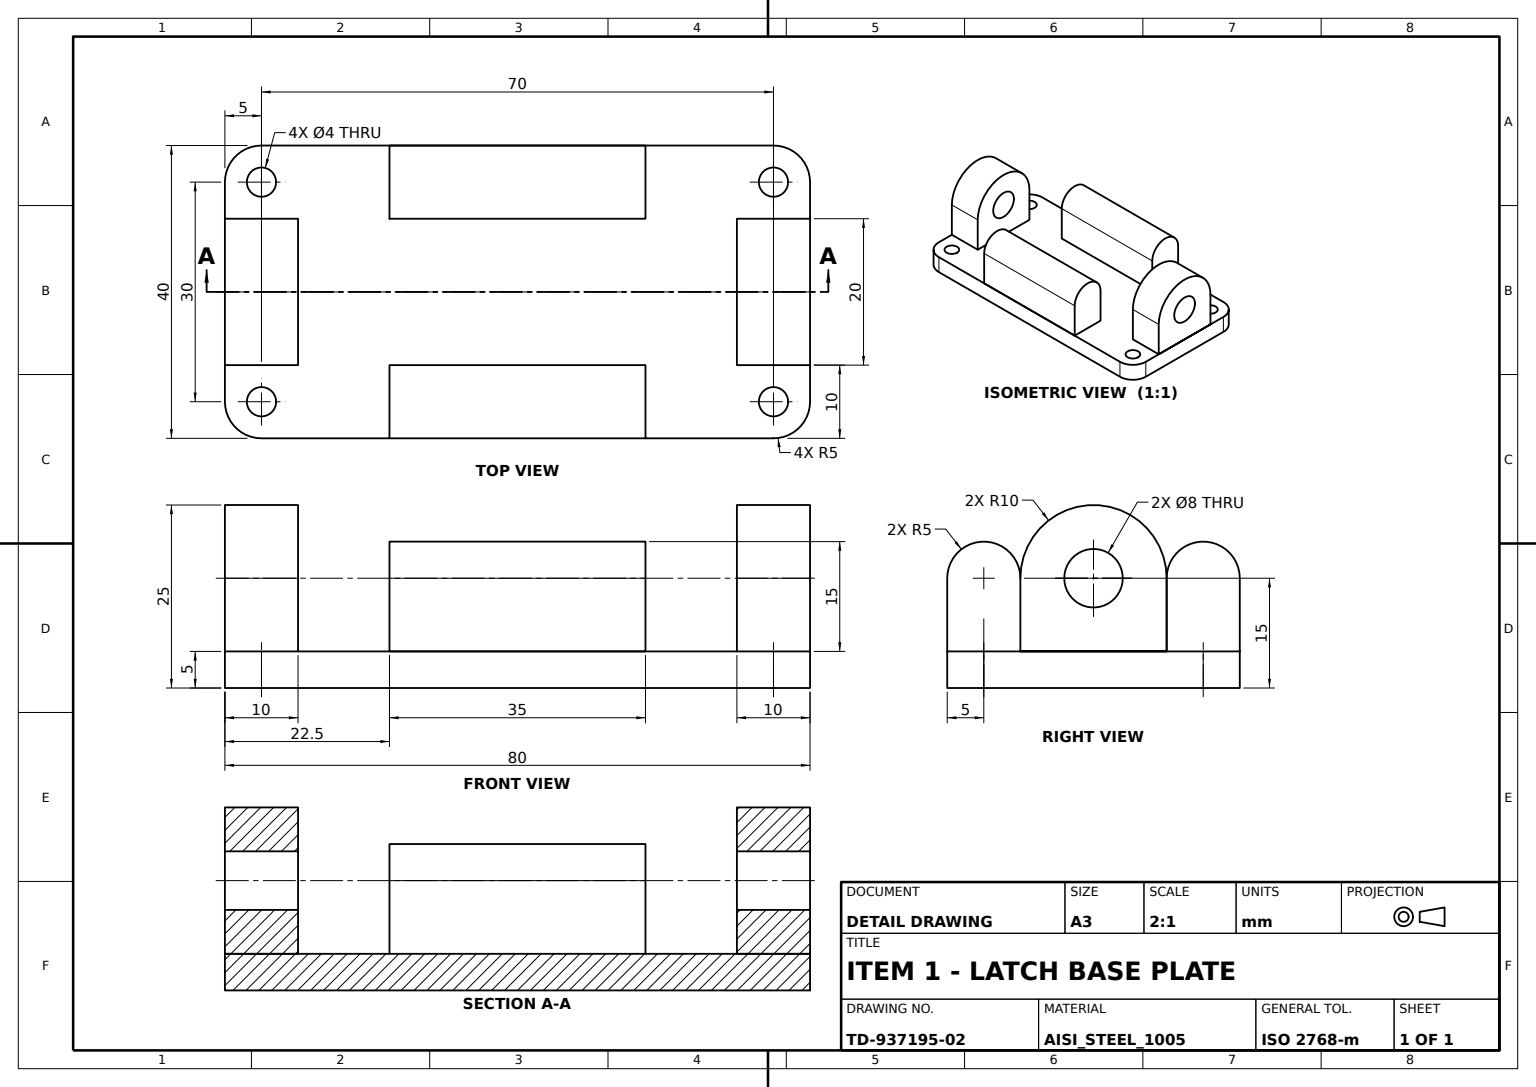
ISO-10303-21;
HEADER;
FILE_DESCRIPTION((''),'2;1');
FILE_NAME('','',(''),(''),'','','');
FILE_SCHEMA(('AUTOMOTIVE_DESIGN'));
ENDSEC;
DATA;
#1=APPLICATION_CONTEXT('');
#2=PRODUCT_CONTEXT('',#1,'mechanical');
#3=PRODUCT('','','',(#2));
#4=PRODUCT_DEFINITION_FORMATION('','',#3);
#5=PRODUCT_DEFINITION_CONTEXT('',#1,'design');
#6=PRODUCT_DEFINITION('','',#4,#5);
#7=PRODUCT_DEFINITION_SHAPE('','',#6);
#8=(LENGTH_UNIT()NAMED_UNIT(*)SI_UNIT(.MILLI.,.METRE.));
#9=(NAMED_UNIT(*)PLANE_ANGLE_UNIT()SI_UNIT($,.RADIAN.));
#10=(NAMED_UNIT(*)SI_UNIT($,.STERADIAN.)SOLID_ANGLE_UNIT());
#11=UNCERTAINTY_MEASURE_WITH_UNIT(LENGTH_MEASURE(0.005),#8,'distance_accuracy_value','');
#12=(GEOMETRIC_REPRESENTATION_CONTEXT(3)GLOBAL_UNCERTAINTY_ASSIGNED_CONTEXT((#11))GLOBAL_UNIT_ASSIGNED_CONTEXT((#8,#9,#10))REPRESENTATION_CONTEXT('',''));
#13=CARTESIAN_POINT('',(-17.5,10.,5.));
#14=VERTEX_POINT('',#13);
#15=CARTESIAN_POINT('',(17.5,10.,5.));
#16=VERTEX_POINT('',#15);
#17=DIRECTION('',(-1.,0.,0.));
#18=VECTOR('',#17,1000.);
#19=LINE('',#15,#18);
#20=EDGE_CURVE('',#14,#16,#19,.F.);
#21=ORIENTED_EDGE('',*,*,#20,.T.);
#22=CARTESIAN_POINT('',(17.5,10.,15.));
#23=VERTEX_POINT('',#22);
#24=CARTESIAN_POINT('',(17.5,10.,20.));
#25=DIRECTION('',(0.,0.,-1.));
#26=VECTOR('',#25,1000.);
#27=LINE('',#24,#26);
#28=EDGE_CURVE('',#16,#23,#27,.F.);
#29=ORIENTED_EDGE('',*,*,#28,.T.);
#30=CARTESIAN_POINT('',(-17.5,10.,15.));
#31=VERTEX_POINT('',#30);
#32=CARTESIAN_POINT('',(-20.5,10.,15.));
#33=DIRECTION('',(1.,0.,0.));
#34=VECTOR('',#33,1000.);
#35=LINE('',#32,#34);
#36=EDGE_CURVE('',#31,#23,#35,.T.);
#37=ORIENTED_EDGE('',*,*,#36,.F.);
#38=DIRECTION('',(0.,0.,1.));
#39=VECTOR('',#38,1000.);
#40=LINE('',#13,#39);
#41=EDGE_CURVE('',#31,#14,#40,.F.);
#42=ORIENTED_EDGE('',*,*,#41,.T.);
#43=EDGE_LOOP('',(#21,#29,#37,#42));
#44=FACE_BOUND('',#43,.T.);
#45=CARTESIAN_POINT('',(0.,10.,0.));
#46=DIRECTION('',(0.,1.,0.));
#47=AXIS2_PLACEMENT_3D('',#45,#46,#38);
#48=PLANE('',#47);
#49=ADVANCED_FACE('',(#44),#48,.F.);
#50=CARTESIAN_POINT('',(-17.5,20.,15.));
#51=VERTEX_POINT('',#50);
#52=CARTESIAN_POINT('',(17.5,20.,15.));
#53=VERTEX_POINT('',#52);
#54=CARTESIAN_POINT('',(-20.5,20.,15.));
#55=LINE('',#54,#34);
#56=EDGE_CURVE('',#51,#53,#55,.T.);
#57=ORIENTED_EDGE('',*,*,#56,.F.);
#58=CARTESIAN_POINT('',(-17.5,15.,15.));
#59=AXIS2_PLACEMENT_3D('',#58,#17,#38);
#60=CIRCLE('',#59,5.);
#61=EDGE_CURVE('',#31,#51,#60,.T.);
#62=ORIENTED_EDGE('',*,*,#61,.F.);
#63=ORIENTED_EDGE('',*,*,#36,.T.);
#64=CARTESIAN_POINT('',(17.5,15.,15.));
#65=DIRECTION('',(0.,-1.,0.));
#66=AXIS2_PLACEMENT_3D('',#64,#33,#65);
#67=CIRCLE('',#66,5.);
#68=EDGE_CURVE('',#53,#23,#67,.T.);
#69=ORIENTED_EDGE('',*,*,#68,.F.);
#70=EDGE_LOOP('',(#57,#62,#63,#69));
#71=FACE_BOUND('',#70,.T.);
#72=CARTESIAN_POINT('',(-20.5,15.,15.));
#73=AXIS2_PLACEMENT_3D('',#72,#33,#25);
#74=CYLINDRICAL_SURFACE('',#73,5.);
#75=ADVANCED_FACE('',(#71),#74,.T.);
#76=CARTESIAN_POINT('',(-17.5,20.,5.));
#77=VERTEX_POINT('',#76);
#78=VECTOR('',#46,1000.);
#79=LINE('',#13,#78);
#80=EDGE_CURVE('',#14,#77,#79,.T.);
#81=ORIENTED_EDGE('',*,*,#80,.T.);
#82=CARTESIAN_POINT('',(17.5,20.,5.));
#83=VERTEX_POINT('',#82);
#84=LINE('',#82,#18);
#85=EDGE_CURVE('',#77,#83,#84,.F.);
#86=ORIENTED_EDGE('',*,*,#85,.T.);
#87=LINE('',#15,#78);
#88=EDGE_CURVE('',#16,#83,#87,.T.);
#89=ORIENTED_EDGE('',*,*,#88,.F.);
#90=ORIENTED_EDGE('',*,*,#20,.F.);
#91=EDGE_LOOP('',(#81,#86,#89,#90));
#92=FACE_BOUND('',#91,.T.);
#93=AXIS2_PLACEMENT_3D('',#15,#25,#17);
#94=PLANE('',#93);
#95=ADVANCED_FACE('',(#92),#94,.T.);
#96=ORIENTED_EDGE('',*,*,#80,.F.);
#97=ORIENTED_EDGE('',*,*,#41,.F.);
#98=ORIENTED_EDGE('',*,*,#61,.T.);
#99=LINE('',#76,#39);
#100=EDGE_CURVE('',#51,#77,#99,.F.);
#101=ORIENTED_EDGE('',*,*,#100,.T.);
#102=EDGE_LOOP('',(#96,#97,#98,#101));
#103=FACE_BOUND('',#102,.T.);
#104=AXIS2_PLACEMENT_3D('',#13,#17,#38);
#105=PLANE('',#104);
#106=ADVANCED_FACE('',(#103),#105,.T.);
#107=ORIENTED_EDGE('',*,*,#88,.T.);
#108=CARTESIAN_POINT('',(17.5,20.,20.));
#109=LINE('',#108,#26);
#110=EDGE_CURVE('',#83,#53,#109,.F.);
#111=ORIENTED_EDGE('',*,*,#110,.T.);
#112=ORIENTED_EDGE('',*,*,#68,.T.);
#113=ORIENTED_EDGE('',*,*,#28,.F.);
#114=EDGE_LOOP('',(#107,#111,#112,#113));
#115=FACE_BOUND('',#114,.T.);
#116=AXIS2_PLACEMENT_3D('',#24,#33,#25);
#117=PLANE('',#116);
#118=ADVANCED_FACE('',(#115),#117,.T.);
#119=ORIENTED_EDGE('',*,*,#100,.F.);
#120=ORIENTED_EDGE('',*,*,#56,.T.);
#121=ORIENTED_EDGE('',*,*,#110,.F.);
#122=ORIENTED_EDGE('',*,*,#85,.F.);
#123=EDGE_LOOP('',(#119,#120,#121,#122));
#124=FACE_BOUND('',#123,.T.);
#125=CARTESIAN_POINT('',(0.,20.,0.));
#126=AXIS2_PLACEMENT_3D('',#125,#46,#38);
#127=PLANE('',#126);
#128=ADVANCED_FACE('',(#124),#127,.T.);
#129=CLOSED_SHELL('',(#49,#75,#95,#106,#118,#128));
#130=MANIFOLD_SOLID_BREP('',#129);
#131=CARTESIAN_POINT('',(30.,4.,15.000001));
#132=VERTEX_POINT('',#131);
#133=CARTESIAN_POINT('',(30.,0.,15.000001));
#134=AXIS2_PLACEMENT_3D('',#133,#17,#46);
#135=CIRCLE('',#134,4.);
#136=EDGE_CURVE('',#132,#132,#135,.T.);
#137=ORIENTED_EDGE('',*,*,#136,.F.);
#138=EDGE_LOOP('',(#137));
#139=FACE_BOUND('',#138,.T.);
#140=CARTESIAN_POINT('',(30.,10.,15.000001));
#141=VERTEX_POINT('',#140);
#142=CARTESIAN_POINT('',(30.,-10.,15.000001));
#143=VERTEX_POINT('',#142);
#144=AXIS2_PLACEMENT_3D('',#133,#33,#46);
#145=CIRCLE('',#144,10.);
#146=EDGE_CURVE('',#141,#143,#145,.T.);
#147=ORIENTED_EDGE('',*,*,#146,.F.);
#148=CARTESIAN_POINT('',(30.,10.,5.));
#149=VERTEX_POINT('',#148);
#150=LINE('',#148,#39);
#151=EDGE_CURVE('',#149,#141,#150,.T.);
#152=ORIENTED_EDGE('',*,*,#151,.F.);
#153=CARTESIAN_POINT('',(30.,-10.,5.));
#154=VERTEX_POINT('',#153);
#155=LINE('',#153,#78);
#156=EDGE_CURVE('',#154,#149,#155,.T.);
#157=ORIENTED_EDGE('',*,*,#156,.F.);
#158=LINE('',#142,#26);
#159=EDGE_CURVE('',#143,#154,#158,.T.);
#160=ORIENTED_EDGE('',*,*,#159,.F.);
#161=EDGE_LOOP('',(#147,#152,#157,#160));
#162=FACE_BOUND('',#161,.T.);
#163=AXIS2_PLACEMENT_3D('',#133,#33,#25);
#164=PLANE('',#163);
#165=ADVANCED_FACE('',(#139,#162),#164,.F.);
#166=ORIENTED_EDGE('',*,*,#146,.T.);
#167=CARTESIAN_POINT('',(40.,-10.,15.000001));
#168=VERTEX_POINT('',#167);
#169=LINE('',#142,#34);
#170=EDGE_CURVE('',#143,#168,#169,.T.);
#171=ORIENTED_EDGE('',*,*,#170,.T.);
#172=CARTESIAN_POINT('',(40.,10.,15.000001));
#173=VERTEX_POINT('',#172);
#174=CARTESIAN_POINT('',(40.,0.,15.000001));
#175=AXIS2_PLACEMENT_3D('',#174,#33,#46);
#176=CIRCLE('',#175,10.);
#177=EDGE_CURVE('',#173,#168,#176,.T.);
#178=ORIENTED_EDGE('',*,*,#177,.F.);
#179=LINE('',#140,#34);
#180=EDGE_CURVE('',#141,#173,#179,.T.);
#181=ORIENTED_EDGE('',*,*,#180,.F.);
#182=EDGE_LOOP('',(#166,#171,#178,#181));
#183=FACE_BOUND('',#182,.T.);
#184=CYLINDRICAL_SURFACE('',#163,10.);
#185=ADVANCED_FACE('',(#183),#184,.T.);
#186=CARTESIAN_POINT('',(40.,-10.,5.));
#187=VERTEX_POINT('',#186);
#188=LINE('',#153,#34);
#189=EDGE_CURVE('',#154,#187,#188,.T.);
#190=ORIENTED_EDGE('',*,*,#189,.T.);
#191=LINE('',#167,#26);
#192=EDGE_CURVE('',#168,#187,#191,.T.);
#193=ORIENTED_EDGE('',*,*,#192,.F.);
#194=ORIENTED_EDGE('',*,*,#170,.F.);
#195=ORIENTED_EDGE('',*,*,#159,.T.);
#196=EDGE_LOOP('',(#190,#193,#194,#195));
#197=FACE_BOUND('',#196,.T.);
#198=AXIS2_PLACEMENT_3D('',#142,#65,#25);
#199=PLANE('',#198);
#200=ADVANCED_FACE('',(#197),#199,.T.);
#201=ORIENTED_EDGE('',*,*,#136,.T.);
#202=EDGE_LOOP('',(#201));
#203=FACE_BOUND('',#202,.T.);
#204=CARTESIAN_POINT('',(40.,4.,15.000001));
#205=VERTEX_POINT('',#204);
#206=AXIS2_PLACEMENT_3D('',#174,#17,#46);
#207=CIRCLE('',#206,4.);
#208=EDGE_CURVE('',#205,#205,#207,.T.);
#209=ORIENTED_EDGE('',*,*,#208,.F.);
#210=EDGE_LOOP('',(#209));
#211=FACE_BOUND('',#210,.T.);
#212=CYLINDRICAL_SURFACE('',#163,4.);
#213=ADVANCED_FACE('',(#203,#211),#212,.F.);
#214=CARTESIAN_POINT('',(40.,10.,5.));
#215=VERTEX_POINT('',#214);
#216=LINE('',#186,#78);
#217=EDGE_CURVE('',#187,#215,#216,.T.);
#218=ORIENTED_EDGE('',*,*,#217,.F.);
#219=ORIENTED_EDGE('',*,*,#189,.F.);
#220=ORIENTED_EDGE('',*,*,#156,.T.);
#221=LINE('',#148,#34);
#222=EDGE_CURVE('',#149,#215,#221,.T.);
#223=ORIENTED_EDGE('',*,*,#222,.T.);
#224=EDGE_LOOP('',(#218,#219,#220,#223));
#225=FACE_BOUND('',#224,.T.);
#226=AXIS2_PLACEMENT_3D('',#153,#25,#17);
#227=PLANE('',#226);
#228=ADVANCED_FACE('',(#225),#227,.T.);
#229=ORIENTED_EDGE('',*,*,#222,.F.);
#230=ORIENTED_EDGE('',*,*,#151,.T.);
#231=ORIENTED_EDGE('',*,*,#180,.T.);
#232=LINE('',#214,#39);
#233=EDGE_CURVE('',#215,#173,#232,.T.);
#234=ORIENTED_EDGE('',*,*,#233,.F.);
#235=EDGE_LOOP('',(#229,#230,#231,#234));
#236=FACE_BOUND('',#235,.T.);
#237=AXIS2_PLACEMENT_3D('',#148,#46,#38);
#238=PLANE('',#237);
#239=ADVANCED_FACE('',(#236),#238,.T.);
#240=ORIENTED_EDGE('',*,*,#208,.T.);
#241=EDGE_LOOP('',(#240));
#242=FACE_BOUND('',#241,.T.);
#243=ORIENTED_EDGE('',*,*,#217,.T.);
#244=ORIENTED_EDGE('',*,*,#233,.T.);
#245=ORIENTED_EDGE('',*,*,#177,.T.);
#246=ORIENTED_EDGE('',*,*,#192,.T.);
#247=EDGE_LOOP('',(#243,#244,#245,#246));
#248=FACE_BOUND('',#247,.T.);
#249=AXIS2_PLACEMENT_3D('',#174,#33,#25);
#250=PLANE('',#249);
#251=ADVANCED_FACE('',(#242,#248),#250,.T.);
#252=CLOSED_SHELL('',(#165,#185,#200,#213,#228,#239,#251));
#253=MANIFOLD_SOLID_BREP('',#252);
#254=CARTESIAN_POINT('',(17.5,-10.,5.));
#255=VERTEX_POINT('',#254);
#256=CARTESIAN_POINT('',(17.5,-20.,5.));
#257=VERTEX_POINT('',#256);
#258=VECTOR('',#65,1000.);
#259=LINE('',#254,#258);
#260=EDGE_CURVE('',#255,#257,#259,.T.);
#261=ORIENTED_EDGE('',*,*,#260,.T.);
#262=CARTESIAN_POINT('',(-17.5,-20.,5.));
#263=VERTEX_POINT('',#262);
#264=LINE('',#262,#34);
#265=EDGE_CURVE('',#263,#257,#264,.T.);
#266=ORIENTED_EDGE('',*,*,#265,.F.);
#267=CARTESIAN_POINT('',(-17.5,-10.,5.));
#268=VERTEX_POINT('',#267);
#269=LINE('',#267,#258);
#270=EDGE_CURVE('',#268,#263,#269,.T.);
#271=ORIENTED_EDGE('',*,*,#270,.F.);
#272=LINE('',#267,#34);
#273=EDGE_CURVE('',#268,#255,#272,.T.);
#274=ORIENTED_EDGE('',*,*,#273,.T.);
#275=EDGE_LOOP('',(#261,#266,#271,#274));
#276=FACE_BOUND('',#275,.T.);
#277=AXIS2_PLACEMENT_3D('',#267,#25,#17);
#278=PLANE('',#277);
#279=ADVANCED_FACE('',(#276),#278,.T.);
#280=CARTESIAN_POINT('',(17.5,-20.,15.));
#281=VERTEX_POINT('',#280);
#282=CARTESIAN_POINT('',(17.5,-10.,15.));
#283=VERTEX_POINT('',#282);
#284=CARTESIAN_POINT('',(17.5,-15.,15.));
#285=AXIS2_PLACEMENT_3D('',#284,#17,#46);
#286=CIRCLE('',#285,5.);
#287=EDGE_CURVE('',#281,#283,#286,.T.);
#288=ORIENTED_EDGE('',*,*,#287,.T.);
#289=CARTESIAN_POINT('',(-17.5,-10.,15.));
#290=VERTEX_POINT('',#289);
#291=CARTESIAN_POINT('',(-20.5,-10.,15.));
#292=LINE('',#291,#34);
#293=EDGE_CURVE('',#290,#283,#292,.T.);
#294=ORIENTED_EDGE('',*,*,#293,.F.);
#295=CARTESIAN_POINT('',(-17.5,-20.,15.));
#296=VERTEX_POINT('',#295);
#297=CARTESIAN_POINT('',(-17.5,-15.,15.));
#298=AXIS2_PLACEMENT_3D('',#297,#17,#38);
#299=CIRCLE('',#298,5.);
#300=EDGE_CURVE('',#290,#296,#299,.F.);
#301=ORIENTED_EDGE('',*,*,#300,.T.);
#302=CARTESIAN_POINT('',(-20.5,-20.,15.));
#303=LINE('',#302,#34);
#304=EDGE_CURVE('',#296,#281,#303,.T.);
#305=ORIENTED_EDGE('',*,*,#304,.T.);
#306=EDGE_LOOP('',(#288,#294,#301,#305));
#307=FACE_BOUND('',#306,.T.);
#308=CARTESIAN_POINT('',(-20.5,-15.,15.));
#309=AXIS2_PLACEMENT_3D('',#308,#33,#25);
#310=CYLINDRICAL_SURFACE('',#309,5.);
#311=ADVANCED_FACE('',(#307),#310,.T.);
#312=LINE('',#254,#39);
#313=EDGE_CURVE('',#255,#283,#312,.T.);
#314=ORIENTED_EDGE('',*,*,#313,.T.);
#315=ORIENTED_EDGE('',*,*,#287,.F.);
#316=LINE('',#256,#39);
#317=EDGE_CURVE('',#257,#281,#316,.T.);
#318=ORIENTED_EDGE('',*,*,#317,.F.);
#319=ORIENTED_EDGE('',*,*,#260,.F.);
#320=EDGE_LOOP('',(#314,#315,#318,#319));
#321=FACE_BOUND('',#320,.T.);
#322=AXIS2_PLACEMENT_3D('',#254,#33,#25);
#323=PLANE('',#322);
#324=ADVANCED_FACE('',(#321),#323,.T.);
#325=ORIENTED_EDGE('',*,*,#273,.F.);
#326=CARTESIAN_POINT('',(-17.5,-10.,20.));
#327=LINE('',#326,#26);
#328=EDGE_CURVE('',#290,#268,#327,.T.);
#329=ORIENTED_EDGE('',*,*,#328,.F.);
#330=ORIENTED_EDGE('',*,*,#293,.T.);
#331=ORIENTED_EDGE('',*,*,#313,.F.);
#332=EDGE_LOOP('',(#325,#329,#330,#331));
#333=FACE_BOUND('',#332,.T.);
#334=CARTESIAN_POINT('',(0.,-10.,0.));
#335=AXIS2_PLACEMENT_3D('',#334,#65,#25);
#336=PLANE('',#335);
#337=ADVANCED_FACE('',(#333),#336,.F.);
#338=ORIENTED_EDGE('',*,*,#328,.T.);
#339=ORIENTED_EDGE('',*,*,#270,.T.);
#340=CARTESIAN_POINT('',(-17.5,-20.,20.));
#341=LINE('',#340,#26);
#342=EDGE_CURVE('',#296,#263,#341,.T.);
#343=ORIENTED_EDGE('',*,*,#342,.F.);
#344=ORIENTED_EDGE('',*,*,#300,.F.);
#345=EDGE_LOOP('',(#338,#339,#343,#344));
#346=FACE_BOUND('',#345,.T.);
#347=AXIS2_PLACEMENT_3D('',#326,#17,#38);
#348=PLANE('',#347);
#349=ADVANCED_FACE('',(#346),#348,.T.);
#350=ORIENTED_EDGE('',*,*,#265,.T.);
#351=ORIENTED_EDGE('',*,*,#317,.T.);
#352=ORIENTED_EDGE('',*,*,#304,.F.);
#353=ORIENTED_EDGE('',*,*,#342,.T.);
#354=EDGE_LOOP('',(#350,#351,#352,#353));
#355=FACE_BOUND('',#354,.T.);
#356=CARTESIAN_POINT('',(0.,-20.,0.));
#357=AXIS2_PLACEMENT_3D('',#356,#65,#25);
#358=PLANE('',#357);
#359=ADVANCED_FACE('',(#355),#358,.T.);
#360=CLOSED_SHELL('',(#279,#311,#324,#337,#349,#359));
#361=MANIFOLD_SOLID_BREP('',#360);
#362=CARTESIAN_POINT('',(37.,-15.,0.));
#363=VERTEX_POINT('',#362);
#364=CARTESIAN_POINT('',(35.,-15.,0.));
#365=AXIS2_PLACEMENT_3D('',#364,#38,#33);
#366=CIRCLE('',#365,2.);
#367=EDGE_CURVE('',#363,#363,#366,.T.);
#368=ORIENTED_EDGE('',*,*,#367,.F.);
#369=EDGE_LOOP('',(#368));
#370=FACE_BOUND('',#369,.T.);
#371=CARTESIAN_POINT('',(37.,-15.,5.));
#372=VERTEX_POINT('',#371);
#373=CARTESIAN_POINT('',(35.,-15.,5.));
#374=AXIS2_PLACEMENT_3D('',#373,#38,#33);
#375=CIRCLE('',#374,2.);
#376=EDGE_CURVE('',#372,#372,#375,.T.);
#377=ORIENTED_EDGE('',*,*,#376,.T.);
#378=EDGE_LOOP('',(#377));
#379=FACE_BOUND('',#378,.T.);
#380=AXIS2_PLACEMENT_3D('',#373,#25,#17);
#381=CYLINDRICAL_SURFACE('',#380,2.);
#382=ADVANCED_FACE('',(#370,#379),#381,.F.);
#383=CARTESIAN_POINT('',(37.,15.,5.));
#384=VERTEX_POINT('',#383);
#385=CARTESIAN_POINT('',(35.,15.,5.));
#386=AXIS2_PLACEMENT_3D('',#385,#38,#33);
#387=CIRCLE('',#386,2.);
#388=EDGE_CURVE('',#384,#384,#387,.T.);
#389=ORIENTED_EDGE('',*,*,#388,.T.);
#390=EDGE_LOOP('',(#389));
#391=FACE_BOUND('',#390,.T.);
#392=CARTESIAN_POINT('',(37.,15.,0.));
#393=VERTEX_POINT('',#392);
#394=CARTESIAN_POINT('',(35.,15.,0.));
#395=AXIS2_PLACEMENT_3D('',#394,#38,#33);
#396=CIRCLE('',#395,2.);
#397=EDGE_CURVE('',#393,#393,#396,.T.);
#398=ORIENTED_EDGE('',*,*,#397,.F.);
#399=EDGE_LOOP('',(#398));
#400=FACE_BOUND('',#399,.T.);
#401=AXIS2_PLACEMENT_3D('',#385,#25,#17);
#402=CYLINDRICAL_SURFACE('',#401,2.);
#403=ADVANCED_FACE('',(#391,#400),#402,.F.);
#404=CARTESIAN_POINT('',(40.,15.,5.));
#405=VERTEX_POINT('',#404);
#406=CARTESIAN_POINT('',(40.,-15.,5.));
#407=VERTEX_POINT('',#406);
#408=LINE('',#404,#258);
#409=EDGE_CURVE('',#405,#407,#408,.T.);
#410=ORIENTED_EDGE('',*,*,#409,.T.);
#411=CARTESIAN_POINT('',(40.,-15.,0.));
#412=VERTEX_POINT('',#411);
#413=LINE('',#406,#26);
#414=EDGE_CURVE('',#407,#412,#413,.T.);
#415=ORIENTED_EDGE('',*,*,#414,.T.);
#416=CARTESIAN_POINT('',(40.,15.,0.));
#417=VERTEX_POINT('',#416);
#418=LINE('',#416,#258);
#419=EDGE_CURVE('',#417,#412,#418,.T.);
#420=ORIENTED_EDGE('',*,*,#419,.F.);
#421=LINE('',#404,#26);
#422=EDGE_CURVE('',#405,#417,#421,.T.);
#423=ORIENTED_EDGE('',*,*,#422,.F.);
#424=EDGE_LOOP('',(#410,#415,#420,#423));
#425=FACE_BOUND('',#424,.T.);
#426=AXIS2_PLACEMENT_3D('',#404,#33,#25);
#427=PLANE('',#426);
#428=ADVANCED_FACE('',(#425),#427,.T.);
#429=CARTESIAN_POINT('',(-40.,-15.,0.));
#430=VERTEX_POINT('',#429);
#431=CARTESIAN_POINT('',(-40.,15.,0.));
#432=VERTEX_POINT('',#431);
#433=LINE('',#429,#78);
#434=EDGE_CURVE('',#430,#432,#433,.T.);
#435=ORIENTED_EDGE('',*,*,#434,.F.);
#436=CARTESIAN_POINT('',(-40.,-15.,5.));
#437=VERTEX_POINT('',#436);
#438=LINE('',#436,#26);
#439=EDGE_CURVE('',#437,#430,#438,.T.);
#440=ORIENTED_EDGE('',*,*,#439,.F.);
#441=CARTESIAN_POINT('',(-40.,15.,5.));
#442=VERTEX_POINT('',#441);
#443=LINE('',#436,#78);
#444=EDGE_CURVE('',#437,#442,#443,.T.);
#445=ORIENTED_EDGE('',*,*,#444,.T.);
#446=LINE('',#441,#26);
#447=EDGE_CURVE('',#442,#432,#446,.T.);
#448=ORIENTED_EDGE('',*,*,#447,.T.);
#449=EDGE_LOOP('',(#435,#440,#445,#448));
#450=FACE_BOUND('',#449,.T.);
#451=AXIS2_PLACEMENT_3D('',#436,#17,#38);
#452=PLANE('',#451);
#453=ADVANCED_FACE('',(#450),#452,.T.);
#454=CARTESIAN_POINT('',(-33.,-15.,5.));
#455=VERTEX_POINT('',#454);
#456=CARTESIAN_POINT('',(-35.,-15.,5.));
#457=AXIS2_PLACEMENT_3D('',#456,#38,#33);
#458=CIRCLE('',#457,2.);
#459=EDGE_CURVE('',#455,#455,#458,.T.);
#460=ORIENTED_EDGE('',*,*,#459,.T.);
#461=EDGE_LOOP('',(#460));
#462=FACE_BOUND('',#461,.T.);
#463=CARTESIAN_POINT('',(-33.,-15.,0.));
#464=VERTEX_POINT('',#463);
#465=CARTESIAN_POINT('',(-35.,-15.,0.));
#466=AXIS2_PLACEMENT_3D('',#465,#38,#33);
#467=CIRCLE('',#466,2.);
#468=EDGE_CURVE('',#464,#464,#467,.T.);
#469=ORIENTED_EDGE('',*,*,#468,.F.);
#470=EDGE_LOOP('',(#469));
#471=FACE_BOUND('',#470,.T.);
#472=AXIS2_PLACEMENT_3D('',#456,#25,#17);
#473=CYLINDRICAL_SURFACE('',#472,2.);
#474=ADVANCED_FACE('',(#462,#471),#473,.F.);
#475=CARTESIAN_POINT('',(35.,-20.,5.));
#476=VERTEX_POINT('',#475);
#477=CARTESIAN_POINT('',(35.,-20.,0.));
#478=VERTEX_POINT('',#477);
#479=LINE('',#475,#26);
#480=EDGE_CURVE('',#476,#478,#479,.T.);
#481=ORIENTED_EDGE('',*,*,#480,.T.);
#482=AXIS2_PLACEMENT_3D('',#364,#25,#33);
#483=CIRCLE('',#482,5.);
#484=EDGE_CURVE('',#412,#478,#483,.T.);
#485=ORIENTED_EDGE('',*,*,#484,.F.);
#486=ORIENTED_EDGE('',*,*,#414,.F.);
#487=AXIS2_PLACEMENT_3D('',#373,#25,#33);
#488=CIRCLE('',#487,5.);
#489=EDGE_CURVE('',#407,#476,#488,.T.);
#490=ORIENTED_EDGE('',*,*,#489,.T.);
#491=EDGE_LOOP('',(#481,#485,#486,#490));
#492=FACE_BOUND('',#491,.T.);
#493=CYLINDRICAL_SURFACE('',#380,5.);
#494=ADVANCED_FACE('',(#492),#493,.T.);
#495=CARTESIAN_POINT('',(-35.,-20.,5.));
#496=VERTEX_POINT('',#495);
#497=CARTESIAN_POINT('',(-35.,-20.,0.));
#498=VERTEX_POINT('',#497);
#499=LINE('',#495,#26);
#500=EDGE_CURVE('',#496,#498,#499,.T.);
#501=ORIENTED_EDGE('',*,*,#500,.T.);
#502=LINE('',#477,#18);
#503=EDGE_CURVE('',#478,#498,#502,.T.);
#504=ORIENTED_EDGE('',*,*,#503,.F.);
#505=ORIENTED_EDGE('',*,*,#480,.F.);
#506=LINE('',#475,#18);
#507=EDGE_CURVE('',#476,#496,#506,.T.);
#508=ORIENTED_EDGE('',*,*,#507,.T.);
#509=EDGE_LOOP('',(#501,#504,#505,#508));
#510=FACE_BOUND('',#509,.T.);
#511=AXIS2_PLACEMENT_3D('',#475,#65,#25);
#512=PLANE('',#511);
#513=ADVANCED_FACE('',(#510),#512,.T.);
#514=CARTESIAN_POINT('',(-33.,15.,5.));
#515=VERTEX_POINT('',#514);
#516=CARTESIAN_POINT('',(-35.,15.,5.));
#517=AXIS2_PLACEMENT_3D('',#516,#38,#33);
#518=CIRCLE('',#517,2.);
#519=EDGE_CURVE('',#515,#515,#518,.T.);
#520=ORIENTED_EDGE('',*,*,#519,.T.);
#521=EDGE_LOOP('',(#520));
#522=FACE_BOUND('',#521,.T.);
#523=CARTESIAN_POINT('',(-33.,15.,0.));
#524=VERTEX_POINT('',#523);
#525=CARTESIAN_POINT('',(-35.,15.,0.));
#526=AXIS2_PLACEMENT_3D('',#525,#38,#33);
#527=CIRCLE('',#526,2.);
#528=EDGE_CURVE('',#524,#524,#527,.T.);
#529=ORIENTED_EDGE('',*,*,#528,.F.);
#530=EDGE_LOOP('',(#529));
#531=FACE_BOUND('',#530,.T.);
#532=AXIS2_PLACEMENT_3D('',#516,#25,#17);
#533=CYLINDRICAL_SURFACE('',#532,2.);
#534=ADVANCED_FACE('',(#522,#531),#533,.F.);
#535=ORIENTED_EDGE('',*,*,#388,.F.);
#536=EDGE_LOOP('',(#535));
#537=FACE_BOUND('',#536,.T.);
#538=ORIENTED_EDGE('',*,*,#459,.F.);
#539=EDGE_LOOP('',(#538));
#540=FACE_BOUND('',#539,.T.);
#541=ORIENTED_EDGE('',*,*,#376,.F.);
#542=EDGE_LOOP('',(#541));
#543=FACE_BOUND('',#542,.T.);
#544=ORIENTED_EDGE('',*,*,#519,.F.);
#545=EDGE_LOOP('',(#544));
#546=FACE_BOUND('',#545,.T.);
#547=ORIENTED_EDGE('',*,*,#489,.F.);
#548=ORIENTED_EDGE('',*,*,#409,.F.);
#549=CARTESIAN_POINT('',(35.,20.,5.));
#550=VERTEX_POINT('',#549);
#551=AXIS2_PLACEMENT_3D('',#385,#25,#33);
#552=CIRCLE('',#551,5.);
#553=EDGE_CURVE('',#550,#405,#552,.T.);
#554=ORIENTED_EDGE('',*,*,#553,.F.);
#555=CARTESIAN_POINT('',(-35.,20.,5.));
#556=VERTEX_POINT('',#555);
#557=LINE('',#555,#34);
#558=EDGE_CURVE('',#556,#550,#557,.T.);
#559=ORIENTED_EDGE('',*,*,#558,.F.);
#560=AXIS2_PLACEMENT_3D('',#516,#25,#33);
#561=CIRCLE('',#560,5.);
#562=EDGE_CURVE('',#442,#556,#561,.T.);
#563=ORIENTED_EDGE('',*,*,#562,.F.);
#564=ORIENTED_EDGE('',*,*,#444,.F.);
#565=AXIS2_PLACEMENT_3D('',#456,#25,#33);
#566=CIRCLE('',#565,5.);
#567=EDGE_CURVE('',#496,#437,#566,.T.);
#568=ORIENTED_EDGE('',*,*,#567,.F.);
#569=ORIENTED_EDGE('',*,*,#507,.F.);
#570=EDGE_LOOP('',(#547,#548,#554,#559,#563,#564,#568,#569));
#571=FACE_BOUND('',#570,.T.);
#572=PLANE('',#472);
#573=ADVANCED_FACE('',(#537,#540,#543,#546,#571),#572,.F.);
#574=ORIENTED_EDGE('',*,*,#367,.T.);
#575=EDGE_LOOP('',(#574));
#576=FACE_BOUND('',#575,.T.);
#577=ORIENTED_EDGE('',*,*,#528,.T.);
#578=EDGE_LOOP('',(#577));
#579=FACE_BOUND('',#578,.T.);
#580=ORIENTED_EDGE('',*,*,#468,.T.);
#581=EDGE_LOOP('',(#580));
#582=FACE_BOUND('',#581,.T.);
#583=CARTESIAN_POINT('',(-35.,20.,0.));
#584=VERTEX_POINT('',#583);
#585=AXIS2_PLACEMENT_3D('',#525,#25,#33);
#586=CIRCLE('',#585,5.);
#587=EDGE_CURVE('',#432,#584,#586,.T.);
#588=ORIENTED_EDGE('',*,*,#587,.T.);
#589=CARTESIAN_POINT('',(35.,20.,0.));
#590=VERTEX_POINT('',#589);
#591=LINE('',#583,#34);
#592=EDGE_CURVE('',#584,#590,#591,.T.);
#593=ORIENTED_EDGE('',*,*,#592,.T.);
#594=AXIS2_PLACEMENT_3D('',#394,#25,#33);
#595=CIRCLE('',#594,5.);
#596=EDGE_CURVE('',#590,#417,#595,.T.);
#597=ORIENTED_EDGE('',*,*,#596,.T.);
#598=ORIENTED_EDGE('',*,*,#419,.T.);
#599=ORIENTED_EDGE('',*,*,#484,.T.);
#600=ORIENTED_EDGE('',*,*,#503,.T.);
#601=AXIS2_PLACEMENT_3D('',#465,#25,#33);
#602=CIRCLE('',#601,5.);
#603=EDGE_CURVE('',#498,#430,#602,.T.);
#604=ORIENTED_EDGE('',*,*,#603,.T.);
#605=ORIENTED_EDGE('',*,*,#434,.T.);
#606=EDGE_LOOP('',(#588,#593,#597,#598,#599,#600,#604,#605));
#607=FACE_BOUND('',#606,.T.);
#608=ORIENTED_EDGE('',*,*,#397,.T.);
#609=EDGE_LOOP('',(#608));
#610=FACE_BOUND('',#609,.T.);
#611=AXIS2_PLACEMENT_3D('',#465,#25,#17);
#612=PLANE('',#611);
#613=ADVANCED_FACE('',(#576,#579,#582,#607,#610),#612,.T.);
#614=ORIENTED_EDGE('',*,*,#596,.F.);
#615=LINE('',#549,#26);
#616=EDGE_CURVE('',#550,#590,#615,.T.);
#617=ORIENTED_EDGE('',*,*,#616,.F.);
#618=ORIENTED_EDGE('',*,*,#553,.T.);
#619=ORIENTED_EDGE('',*,*,#422,.T.);
#620=EDGE_LOOP('',(#614,#617,#618,#619));
#621=FACE_BOUND('',#620,.T.);
#622=CYLINDRICAL_SURFACE('',#401,5.);
#623=ADVANCED_FACE('',(#621),#622,.T.);
#624=ORIENTED_EDGE('',*,*,#616,.T.);
#625=ORIENTED_EDGE('',*,*,#592,.F.);
#626=LINE('',#555,#26);
#627=EDGE_CURVE('',#556,#584,#626,.T.);
#628=ORIENTED_EDGE('',*,*,#627,.F.);
#629=ORIENTED_EDGE('',*,*,#558,.T.);
#630=EDGE_LOOP('',(#624,#625,#628,#629));
#631=FACE_BOUND('',#630,.T.);
#632=AXIS2_PLACEMENT_3D('',#555,#46,#17);
#633=PLANE('',#632);
#634=ADVANCED_FACE('',(#631),#633,.T.);
#635=ORIENTED_EDGE('',*,*,#447,.F.);
#636=ORIENTED_EDGE('',*,*,#562,.T.);
#637=ORIENTED_EDGE('',*,*,#627,.T.);
#638=ORIENTED_EDGE('',*,*,#587,.F.);
#639=EDGE_LOOP('',(#635,#636,#637,#638));
#640=FACE_BOUND('',#639,.T.);
#641=CYLINDRICAL_SURFACE('',#532,5.);
#642=ADVANCED_FACE('',(#640),#641,.T.);
#643=ORIENTED_EDGE('',*,*,#500,.F.);
#644=ORIENTED_EDGE('',*,*,#567,.T.);
#645=ORIENTED_EDGE('',*,*,#439,.T.);
#646=ORIENTED_EDGE('',*,*,#603,.F.);
#647=EDGE_LOOP('',(#643,#644,#645,#646));
#648=FACE_BOUND('',#647,.T.);
#649=CYLINDRICAL_SURFACE('',#472,5.);
#650=ADVANCED_FACE('',(#648),#649,.T.);
#651=CLOSED_SHELL('',(#382,#403,#428,#453,#474,#494,#513,#534,#573,#613,#623,#634,#642,#650));
#652=MANIFOLD_SOLID_BREP('',#651);
#653=CARTESIAN_POINT('',(-30.,10.,5.));
#654=VERTEX_POINT('',#653);
#655=CARTESIAN_POINT('',(-40.,10.,5.));
#656=VERTEX_POINT('',#655);
#657=LINE('',#653,#18);
#658=EDGE_CURVE('',#654,#656,#657,.T.);
#659=ORIENTED_EDGE('',*,*,#658,.T.);
#660=CARTESIAN_POINT('',(-40.,10.,15.000001));
#661=VERTEX_POINT('',#660);
#662=LINE('',#655,#39);
#663=EDGE_CURVE('',#656,#661,#662,.T.);
#664=ORIENTED_EDGE('',*,*,#663,.T.);
#665=CARTESIAN_POINT('',(-30.,10.,15.000001));
#666=VERTEX_POINT('',#665);
#667=LINE('',#665,#18);
#668=EDGE_CURVE('',#666,#661,#667,.T.);
#669=ORIENTED_EDGE('',*,*,#668,.F.);
#670=LINE('',#653,#39);
#671=EDGE_CURVE('',#654,#666,#670,.T.);
#672=ORIENTED_EDGE('',*,*,#671,.F.);
#673=EDGE_LOOP('',(#659,#664,#669,#672));
#674=FACE_BOUND('',#673,.T.);
#675=AXIS2_PLACEMENT_3D('',#653,#65,#25);
#676=PLANE('',#675);
#677=ADVANCED_FACE('',(#674),#676,.F.);
#678=CARTESIAN_POINT('',(-30.,-10.,15.000001));
#679=VERTEX_POINT('',#678);
#680=CARTESIAN_POINT('',(-30.,-10.,5.));
#681=VERTEX_POINT('',#680);
#682=LINE('',#678,#26);
#683=EDGE_CURVE('',#679,#681,#682,.T.);
#684=ORIENTED_EDGE('',*,*,#683,.F.);
#685=CARTESIAN_POINT('',(-40.,-10.,15.000001));
#686=VERTEX_POINT('',#685);
#687=LINE('',#678,#18);
#688=EDGE_CURVE('',#679,#686,#687,.T.);
#689=ORIENTED_EDGE('',*,*,#688,.T.);
#690=CARTESIAN_POINT('',(-40.,-10.,5.));
#691=VERTEX_POINT('',#690);
#692=LINE('',#685,#26);
#693=EDGE_CURVE('',#686,#691,#692,.T.);
#694=ORIENTED_EDGE('',*,*,#693,.T.);
#695=LINE('',#680,#18);
#696=EDGE_CURVE('',#681,#691,#695,.T.);
#697=ORIENTED_EDGE('',*,*,#696,.F.);
#698=EDGE_LOOP('',(#684,#689,#694,#697));
#699=FACE_BOUND('',#698,.T.);
#700=AXIS2_PLACEMENT_3D('',#678,#46,#38);
#701=PLANE('',#700);
#702=ADVANCED_FACE('',(#699),#701,.F.);
#703=CARTESIAN_POINT('',(-40.,0.,15.000001));
#704=AXIS2_PLACEMENT_3D('',#703,#33,#46);
#705=CIRCLE('',#704,10.);
#706=EDGE_CURVE('',#661,#686,#705,.T.);
#707=ORIENTED_EDGE('',*,*,#706,.T.);
#708=ORIENTED_EDGE('',*,*,#688,.F.);
#709=CARTESIAN_POINT('',(-30.,0.,15.000001));
#710=AXIS2_PLACEMENT_3D('',#709,#33,#46);
#711=CIRCLE('',#710,10.);
#712=EDGE_CURVE('',#666,#679,#711,.T.);
#713=ORIENTED_EDGE('',*,*,#712,.F.);
#714=ORIENTED_EDGE('',*,*,#668,.T.);
#715=EDGE_LOOP('',(#707,#708,#713,#714));
#716=FACE_BOUND('',#715,.T.);
#717=AXIS2_PLACEMENT_3D('',#709,#17,#38);
#718=CYLINDRICAL_SURFACE('',#717,10.);
#719=ADVANCED_FACE('',(#716),#718,.T.);
#720=CARTESIAN_POINT('',(-30.,4.,15.000001));
#721=VERTEX_POINT('',#720);
#722=AXIS2_PLACEMENT_3D('',#709,#17,#46);
#723=CIRCLE('',#722,4.);
#724=EDGE_CURVE('',#721,#721,#723,.T.);
#725=ORIENTED_EDGE('',*,*,#724,.F.);
#726=EDGE_LOOP('',(#725));
#727=FACE_BOUND('',#726,.T.);
#728=CARTESIAN_POINT('',(-40.,4.,15.000001));
#729=VERTEX_POINT('',#728);
#730=AXIS2_PLACEMENT_3D('',#703,#17,#46);
#731=CIRCLE('',#730,4.);
#732=EDGE_CURVE('',#729,#729,#731,.T.);
#733=ORIENTED_EDGE('',*,*,#732,.T.);
#734=EDGE_LOOP('',(#733));
#735=FACE_BOUND('',#734,.T.);
#736=CYLINDRICAL_SURFACE('',#717,4.);
#737=ADVANCED_FACE('',(#727,#735),#736,.F.);
#738=LINE('',#690,#78);
#739=EDGE_CURVE('',#691,#656,#738,.T.);
#740=ORIENTED_EDGE('',*,*,#739,.F.);
#741=ORIENTED_EDGE('',*,*,#693,.F.);
#742=ORIENTED_EDGE('',*,*,#706,.F.);
#743=ORIENTED_EDGE('',*,*,#663,.F.);
#744=EDGE_LOOP('',(#740,#741,#742,#743));
#745=FACE_BOUND('',#744,.T.);
#746=ORIENTED_EDGE('',*,*,#732,.F.);
#747=EDGE_LOOP('',(#746));
#748=FACE_BOUND('',#747,.T.);
#749=AXIS2_PLACEMENT_3D('',#703,#33,#25);
#750=PLANE('',#749);
#751=ADVANCED_FACE('',(#745,#748),#750,.F.);
#752=LINE('',#680,#78);
#753=EDGE_CURVE('',#681,#654,#752,.T.);
#754=ORIENTED_EDGE('',*,*,#753,.T.);
#755=ORIENTED_EDGE('',*,*,#671,.T.);
#756=ORIENTED_EDGE('',*,*,#712,.T.);
#757=ORIENTED_EDGE('',*,*,#683,.T.);
#758=EDGE_LOOP('',(#754,#755,#756,#757));
#759=FACE_BOUND('',#758,.T.);
#760=ORIENTED_EDGE('',*,*,#724,.T.);
#761=EDGE_LOOP('',(#760));
#762=FACE_BOUND('',#761,.T.);
#763=AXIS2_PLACEMENT_3D('',#709,#33,#25);
#764=PLANE('',#763);
#765=ADVANCED_FACE('',(#759,#762),#764,.T.);
#766=ORIENTED_EDGE('',*,*,#753,.F.);
#767=ORIENTED_EDGE('',*,*,#696,.T.);
#768=ORIENTED_EDGE('',*,*,#739,.T.);
#769=ORIENTED_EDGE('',*,*,#658,.F.);
#770=EDGE_LOOP('',(#766,#767,#768,#769));
#771=FACE_BOUND('',#770,.T.);
#772=AXIS2_PLACEMENT_3D('',#680,#38,#33);
#773=PLANE('',#772);
#774=ADVANCED_FACE('',(#771),#773,.F.);
#775=CLOSED_SHELL('',(#677,#702,#719,#737,#751,#765,#774));
#776=MANIFOLD_SOLID_BREP('',#775);
#777=ADVANCED_BREP_SHAPE_REPRESENTATION('',(#130,#253,#361,#652,#776),#12);
#778=SHAPE_DEFINITION_REPRESENTATION(#7,#777);
ENDSEC;
END-ISO-10303-21;
